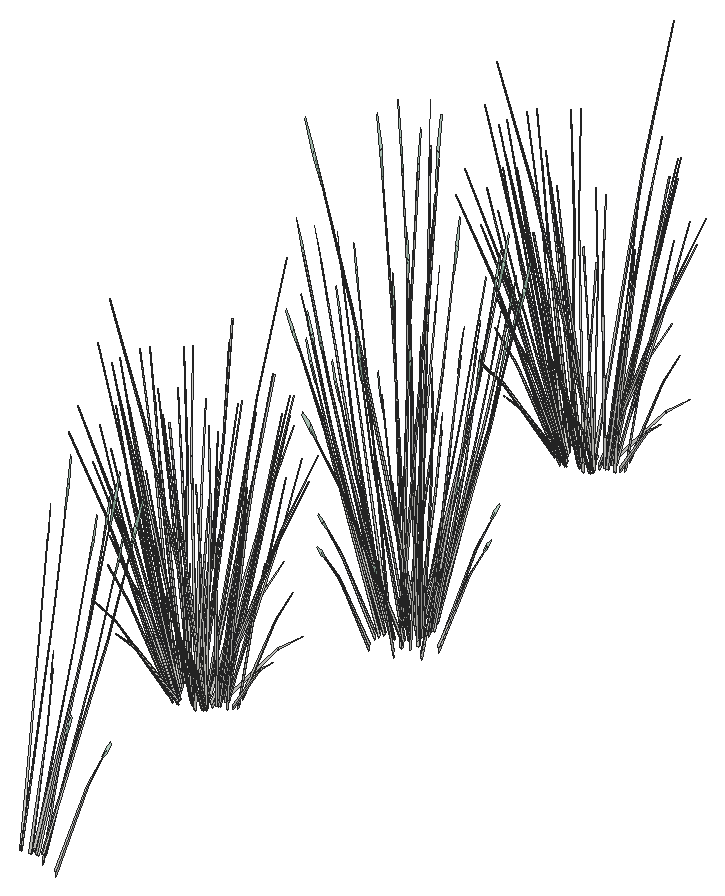
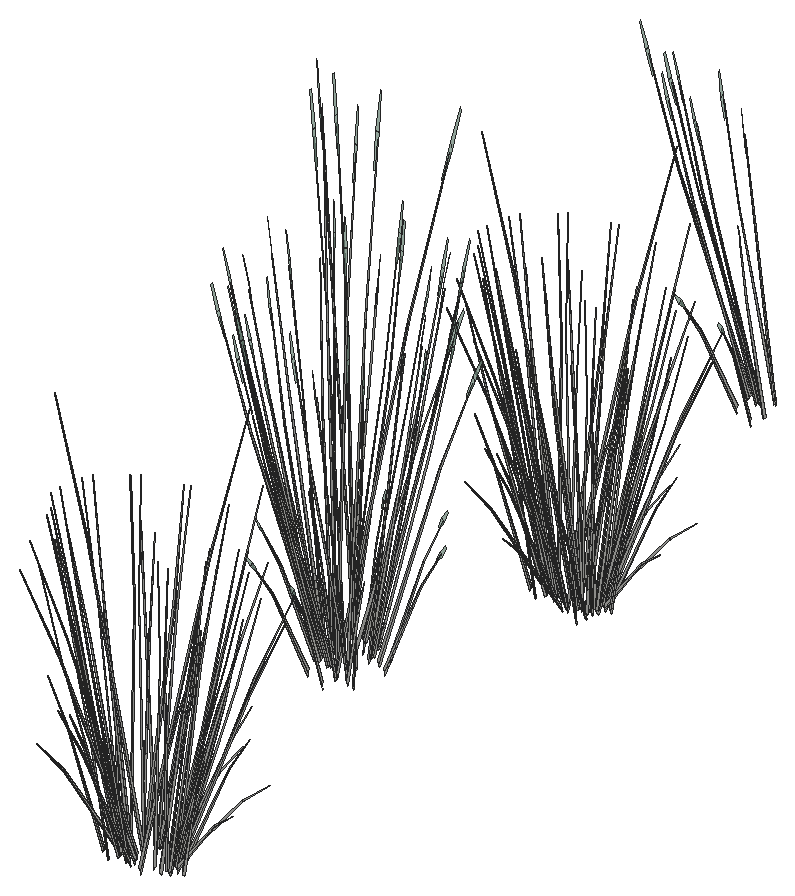
# SketchUp Ruby script. Lengths in inches.
U = 1.inch
M = Sketchup.active_model
def pt(a) = Geom::Point3d.new(a.map { |v| v * U })
def face(e, loops, mat)
  f = e.add_face(loops[0].map { |a| pt(a) })
  loops[1..].each { |l| e.add_face(l.map { |a| pt(a) }).erase! }
  f.material = f.back_material = mat if mat
  f
end
# faces: each face lists its corners as indices into pts; further lists are holes
def faces(e, pts, list, mat = nil) = list.each { |f| face(e, (f[0].is_a?(Array) ? f : [f]).map { |l| l.map { |i| pts[i] } }, mat) }
# xy, xz, yz: faces in a plane at the given z, y or x. An outline is a flat list of corners, or four numbers for a rectangle; further outlines are holes
def ring(l) = l.size == 4 ? [[l[0], l[1]], [l[2], l[1]], [l[2], l[3]], [l[0], l[3]]] : l.each_slice(2).to_a
def flat(e, list, mat, &to3) = list.each { |f| face(e, (f[0].is_a?(Array) ? f : [f]).map { |l| ring(l).map { |u, v| to3.(u, v) } }, mat) }
def xy(e, z, list, mat = nil) = flat(e, list, mat) { |x, y| [x, y, z] }
def xz(e, y, list, mat = nil) = flat(e, list, mat) { |x, z| [x, y, z] }
def yz(e, x, list, mat = nil) = flat(e, list, mat) { |y, z| [x, y, z] }
def lines(e, pts, list) = list.each { |a, b| e.add_line(pt(pts[a]), pt(pts[b])) }
# prism: a flat outline (further loops are holes) pulled along v
def prism(e, loops, v, mat = nil)
  f = face(e, loops, mat); d = Geom::Vector3d.new(v.map { |x| x * U })
  f.pushpull(f.normal.samedirection?(d) ? d.length : -d.length)
end
def box(e, o, s, mat = nil) = prism(e, [[o, [o[0] + s[0], o[1], o[2]], [o[0] + s[0], o[1] + s[1], o[2]], [o[0], o[1] + s[1], o[2]]]], [0, 0, s[2]], mat)
def at(x, y, z, deg = 0) = Geom::Transformation.translation(pt([x, y, z])) * Geom::Transformation.rotation(ORIGIN, Z_AXIS, deg.degrees)
def axes(o, x, y, z) = Geom::Transformation.new([*x, 0, *y, 0, *z, 0, *pt(o).to_a, 1])
def part(name) = M.definitions.add(name)
# library, detail: a bought-in or finely detailed component or shape, given as its bounding box
def library(name, o, s) = part(name).tap { |d| box(d.entities, o, s) }
def detail(e, o, s) = box(e.add_group.entities, o, s)
def put(e, d, t, mat = nil) = e.add_instance(d, t).tap { |i| i.material = mat if mat }
def group(e, t, mat = nil) = e.add_group.tap { |g| g.transformation = t; g.material = mat if mat }.entities
root = M.entities
M.materials.add("LightPink_Translucent").color = [175, 214, 192]
M.materials["LightPink_Translucent"].alpha = 0.75
c1 = part("blade")
p = [[2.15,0.21,22],[0,0.17,0],[0.09,0.45,0],[2.18,0.31,22],[2.29,0.31,22],[0.38,0.45,0],
  [2.48,0.24,33],[2.49,0.24,33],[2.48,0.22,33]]
faces(c1.entities,p,[[0,1,2,3],[4,5,2,3],[6,3,4,7],[8,0,3,6]])
c2 = part("seeds")
p = [[0.3,-0.1,1.38],[-0.01,-0.03,1.59],[-0.01,-0.03,0.03],[0.14,-0.07,-0.07],[0.29,-0.03,3],[0.15,0.01,3.11]]
faces(c2.entities,p,[[0,1,2,3],[1,0,4,5]],"LightPink_Translucent")
c3 = part("blade with seeds")
put(c3.entities,c1,at(0,0,0))
put(c3.entities,c2,axes([2.4,0.25,30.99],[1.5799,-0.05474,1.17369],[-0.12525,1.92788,0.29478],[-0.07173,-0.02425,1.56792]))
c4 = part("blade with seeds\#1")
put(c4.entities,c1,at(0,0,0))
put(root,c3,axes([491.72,471.85,140.75],[0.37435,-0.09148,-0.03177],[0.08606,0.43236,-0.14407],[-0.02373,0.09029,0.47519]))
put(root,c3,axes([494.63,471.6,139.6875],[-0.2267,-0.15919,1.04523],[0.30457,-0.13683,0.76796],[0.07632,0.13148,0.23022]))
put(root,c3,axes([493.78,471.37,141.29],[0.06364,0.41603,-0.32227],[-0.36383,0.10985,0.41605],[0.09772,0.11922,0.79608]))
put(root,c3,axes([493.66,471.04,141.7],[0.35138,0.24965,-0.64651],[-0.24972,0.43748,0.07802],[0.12731,0.14906,0.91455]))
put(root,c3,axes([491.77,471.04,141.29],[-0.27882,0.27194,-0.32227],[-0.26394,-0.31051,0.41605],[-0.04016,0.15777,0.79608]))
put(root,c3,axes([492.92,471.24,141.43],[0.40508,0.12948,-0.465],[-0.13885,0.44393,-0.36018],[0.03714,0.17873,0.88973]))
put(root,c3,axes([492.66,472.36,139.6875],[-0.07352,-0.2953,1.04523],[0.30384,0.139,0.76796],[-0.02079,0.15666,0.23022]))
put(root,c3,axes([492.73,471.52,141.29],[-0.12423,0.3972,-0.32227],[-0.36244,-0.11585,0.41605],[0.03323,0.15992,0.79608]))
put(root,c3,axes([491.95,470.75,141.7],[-0.01072,0.47777,-0.64651],[-0.45152,-0.03209,0.07802],[-0.04765,0.2024,0.91455]))
put(root,c3,axes([492.77,471.16,141.7],[0.19668,0.41997,-0.64651],[-0.40486,0.23405,0.07802],[0.04599,0.20292,0.91455]))
put(root,c4,axes([485.03,499.11,139.9],[0.11364,0.12234,1.40588],[-0.52511,0.103,0.11368],[-0.11868,-0.19206,0.601]))
put(root,c4,axes([485.9,498.29,140.59],[-0.07604,-0.05342,1.43516],[-0.50744,0.03387,-0.22697],[-0.08099,-0.12778,0.1151]))
put(root,c4,axes([488.07,498.68,140.58],[-0.05049,0.0291,1.45516],[-0.49465,-0.09819,-0.1375],[-0.01791,-0.12701,0.25751]))
put(root,c4,axes([488.18,498.95,140.59],[-0.0048,-0.07584,1.43516],[-0.40531,-0.21918,-0.22697],[0.06266,-0.13286,0.1151]))
put(root,c4,axes([486.8,499.32,139.9],[-0.09256,0.13097,1.40588],[-0.38832,-0.27104,0.11368],[0.17518,-0.16893,0.601]))
put(root,c4,axes([486.47,498.93,140.43],[0.14987,-0.29303,-0.29052],[0.43725,0.08547,0.37506],[-0.04009,-0.11798,0.71765]))
put(root,c4,axes([485.375,498.12,140.58],[-0.00927,0.04567,1.45516],[-0.45742,0.16576,-0.1375],[-0.1346,-0.08473,0.25751]))
put(root,c4,axes([486.67,499.12,140.85],[-0.48648,0.17741,-0.09976],[-0.23906,-0.31487,-0.55369],[-0.06419,-0.13269,0.84132]))
put(root,c4,axes([486.53,499,140.6],[0.48986,0.09962,0.39379],[-0.16751,0.3275,0.3247],[-0.02944,-0.12879,0.81485]))
put(root,c4,axes([487.68,499.52,140.85],[-0.54637,-0.01888,-0.09976],[0.01493,-0.35746,-0.55369],[0.03795,-0.13767,0.84132]))
put(root,c4,axes([485.21,499.04,140.43],[-0.07678,-0.30692,-0.29052],[0.43892,-0.08104,0.37506],[-0.11789,-0.08795,0.71765]))
put(root,c4,axes([487.64,499.29,140.43],[0.33637,-0.20062,-0.29052],[0.31842,0.22908,0.37506],[0.04845,-0.11639,0.71765]))
put(root,c4,axes([484.27,499.49,139.9],[0.18466,0.06565,1.40588],[-0.38215,0.27542,0.11368],[-0.23818,-0.12424,0.601]))
put(root,c4,axes([485.5,498.99,141.17],[-0.33178,0.3653,-0.11173],[-0.48049,-0.21045,-0.62013],[-0.16702,-0.10321,0.94228]))
put(root,c4,axes([487.64,499.37,140.6],[0.354,0.25999,0.39379],[-0.37594,0.22422,0.3247],[0.0653,-0.12198,0.81485]))
put(root,c4,axes([484.23,498.88,140.59],[-0.10696,-0.00269,1.43516],[-0.34054,0.26896,-0.22697],[-0.1817,-0.05496,0.1151]))
put(root,c4,axes([488.27,500.22,140.85],[-0.45986,-0.21011,-0.09976],[0.26493,-0.30427,-0.55369],[0.12992,-0.10577,0.84132]))
put(root,c4,axes([489.41,500.13,140.58],[-0.06493,-0.00289,1.45516],[-0.26964,-0.31009,-0.1375],[0.10828,-0.10196,0.25751]))
put(root,c4,axes([486.375,501.37,139.45],[0.4296,0.15365,1.24087],[-0.42086,0.33102,0.4907],[-0.18851,-0.19619,1.04025]))
put(root,c4,axes([484.2,499.58,140.43],[-0.28286,-0.23857,-0.29052],[0.32298,-0.22584,0.37506],[-0.1641,-0.03436,0.71765]))
put(root,c4,axes([488.4,500.01,140.43],[0.43273,-0.05446,-0.29052],[0.11427,0.31131,0.37506],[0.12401,-0.08362,0.71765]))
put(root,c4,axes([488.35,500.08,140.6],[0.12329,0.35069,0.39379],[-0.48364,0.06086,0.3247],[0.14254,-0.08248,0.81485]))
put(root,c4,axes([489.65,500.5,140.59],[0.06898,-0.05804,1.43516],[-0.0883,-0.35603,-0.22697],[0.17309,-0.0675,0.1151]))
put(root,c4,axes([483.82,499.11,140.58],[0.03685,0.03803,1.45516],[-0.17767,0.34183,-0.1375],[-0.17994,0.00247,0.25751]))
put(root,c4,axes([484.52,499.55,140.85],[-0.02662,0.38751,-0.09976],[-0.50399,-0.01059,-0.55369],[-0.19411,-0.02692,0.84132]))
put(root,c4,axes([488.29,501.04,140.85],[-0.25013,-0.34504,-0.09976],[0.44394,-0.16956,-0.55369],[0.18708,-0.04552,0.84132]))
put(root,c4,axes([483.88,500.09,139.9],[0.2062,-0.00863,1.40588],[-0.13679,0.37404,0.11368],[-0.29386,-0.02314,0.601]))
put(root,c4,axes([483.79,500.37,140.6],[0.14045,-0.34743,0.39379],[0.46175,0.1188,0.3247],[-0.18159,0.02088,0.81485]))
put(root,c4,axes([483.7,500.41,140.43],[-0.41315,-0.1063,-0.29052],[0.1205,-0.31012,0.37506],[-0.16634,0.02844,0.71765]))
put(root,c4,axes([488.55,500.9,140.43],[0.41315,0.1063,-0.29052],[-0.1205,0.31012,0.37506],[0.16634,-0.02844,0.71765]))
put(root,c4,axes([487.43,500.52,139.9],[-0.2062,0.00863,1.40588],[0.13679,-0.37404,0.11368],[0.29386,0.02314,0.601]))
put(root,c4,axes([488.46,500.94,140.6],[-0.14045,0.34743,0.39379],[-0.46175,-0.1188,0.3247],[0.18159,-0.02088,0.81485]))
put(root,c4,axes([483.96,500.27,140.85],[0.25013,0.34504,-0.09976],[-0.44394,0.16956,-0.55369],[-0.18708,0.04552,0.84132]))
put(root,c4,axes([489.29,502.07,140.58],[-0.04495,-0.03336,1.45516],[0.09833,-0.35758,-0.1375],[0.17707,-0.02285,0.25751]))
put(root,c4,axes([483.4375,500.61,140.59],[-0.08118,0.04947,1.43516],[0.00691,0.36146,-0.22697],[-0.18608,0.04701,0.1151]))
put(root,c4,axes([488.9,501.77,139.94],[-0.09515,-0.32031,-0.02864],[0.44972,-0.07364,-0.12987],[0.09391,0.02031,0.42837]))
put(root,c4,axes([487.73,501.76,140.85],[0.02662,-0.38751,-0.09976],[0.50399,0.01059,-0.55369],[0.19411,0.02692,0.84132]))
put(root,c4,axes([488.17,501.52,140.59],[0.10664,-0.00644,1.43516],[0.29251,-0.29603,-0.22697],[0.18969,0.03908,0.1151]))
put(root,c4,axes([483.9,501.24,140.6],[-0.12329,-0.35069,0.39379],[0.48364,-0.06086,0.3247],[-0.14254,0.08248,0.81485]))
put(root,c4,axes([483.96,500.75,139.9],[0.17249,-0.0806,1.40588],[0.14522,0.37244,0.11368],[-0.2708,0.08417,0.601]))
put(root,c4,axes([482.53,500.98,140.58],[0.06344,0.01022,1.45516],[0.19627,0.33667,-0.1375],[-0.12987,0.08837,0.25751]))
put(root,c4,axes([483.85,501.3,140.43],[-0.43273,0.05446,-0.29052],[-0.11427,-0.31131,0.37506],[-0.12401,0.08362,0.71765]))
put(root,c4,axes([488.05,501.73,140.43],[0.28286,0.23857,-0.29052],[-0.32298,0.22584,0.37506],[0.1641,0.03436,0.71765]))
put(root,c4,axes([487.94,501.73,140.6],[-0.36656,0.25108,0.39379],[-0.31614,-0.26664,0.3247],[0.17198,0.04631,0.81485]))
put(root,c4,axes([487.07,500.25,140.39],[-0.42958,-0.19798,1.1344],[0.45359,-0.30825,0.48946],[0.1386,0.18577,1.09651]))
put(root,c4,axes([487.04,501.12,139.9],[-0.18466,-0.06565,1.40588],[0.38215,-0.27542,0.11368],[0.23818,0.12424,0.601]))
put(root,c4,axes([483.98,501.09,140.85],[0.45986,0.21011,-0.09976],[-0.26493,0.30427,-0.55369],[-0.12992,0.10577,0.84132]))
put(root,c4,axes([484.6,501,139.9],[0.12417,-0.11708,1.40588],[0.31352,0.31602,0.11368],[-0.21504,0.14392,0.601]))
put(root,c4,axes([486.74,502.18,140.85],[0.29624,-0.32616,-0.09976],[0.42901,0.1879,-0.55369],[0.14913,0.09215,0.84132]))
put(root,c4,axes([486.35,502.45,140.58],[0.00147,-0.04613,1.45516],[0.42603,-0.20353,-0.1375],[0.14798,0.07265,0.25751]))
put(root,c4,axes([484.61,501.95,140.6],[-0.354,-0.25999,0.39379],[0.37594,-0.22422,0.3247],[-0.0653,0.12198,0.81485]))
put(root,c4,axes([486.94,502.23,140.6],[-0.49445,0.08745,0.39379],[-0.08581,-0.34303,0.3247],[0.11629,0.1011,0.81485]))
put(root,c4,axes([484.5,501.28,139.9],[0.09256,-0.13097,1.40588],[0.38832,0.27104,0.11368],[-0.17518,0.16893,0.601]))
put(root,c4,axes([484.61,502.02,140.43],[-0.33637,0.20062,-0.29052],[-0.31842,-0.22908,0.37506],[-0.04845,0.11639,0.71765]))
put(root,c4,axes([483.45,501.96,140.59],[-0.01236,0.0754,1.43516],[0.35069,0.26232,-0.22697],[-0.09181,0.12405,0.1151]))
put(root,c4,axes([484.57,501.79,141.15],[0.54637,0.01888,-0.11073],[-0.01493,0.35746,-0.6146],[-0.03795,0.13767,0.93387]))
put(root,c4,axes([485.58,502.19,140.85],[0.48648,-0.17741,-0.09976],[0.23906,0.31487,-0.55369],[0.06419,0.13269,0.84132]))
put(root,c4,axes([484.94,501.93,140.82],[0.35588,0.25603,-0.4653],[-0.37594,0.22422,-0.36041],[-0.05415,0.13008,0.89031]))
put(root,c4,axes([486.28,501.5,139.9],[-0.11364,-0.12234,1.40588],[0.52511,-0.103,0.11368],[0.11868,0.19206,0.601]))
put(root,c4,axes([485.78,502.38,140.43],[-0.14987,0.29303,-0.29052],[-0.43725,-0.08547,0.37506],[0.04009,0.11798,0.71765]))
put(root,c4,axes([485.35,501.5625,139.9],[-0.01217,-0.14625,1.40588],[0.52737,0.09702,0.11368],[-0.03262,0.20842,0.601]))
put(root,c4,axes([483.41,502.74,140.58],[0.0564,-0.02301,1.45516],[0.46615,0.15302,-0.1375],[-0.01095,0.12741,0.25751]))
put(root,c4,axes([485.47,502.9,140.59],[0.06302,0.06136,1.43516],[0.50855,0.02411,-0.22697],[0.05114,0.13532,0.1151]))
put(root,c4,axes([484.65,502.31,139.48],[0.01092,-0.19671,1.26617],[0.49126,0.1039,0.17497],[-0.04257,0.20964,0.59789]))
put(root,c3,axes([493.37,517.27,140.21],[0.06442,0.13585,1.61128],[-0.4498,0.04685,0.1261],[-0.05969,-0.29426,0.57588]))
put(root,c3,axes([494.09,516.82,141.7],[0.01072,-0.47777,-0.64651],[0.45152,0.03209,0.07802],[0.04765,-0.2024,0.91455]))
put(root,c3,axes([493.3125,516.06,141.29],[0.12423,-0.3972,-0.32227],[0.36244,0.11585,0.41605],[-0.03323,-0.15992,0.79608]))
put(root,c3,axes([493.125,516.33,141.43],[-0.40508,-0.12948,-0.465],[0.13885,-0.44393,-0.36018],[-0.03714,-0.17873,0.88973]))
put(root,c3,axes([494,516.67,141.43],[-0.29499,-0.34704,-0.465],[0.31162,-0.30393,-0.36018],[0.04488,-0.17633,0.88973]))
put(root,c3,axes([491.39,515.45,139.6875],[0.20183,0.19918,1.04523],[-0.31952,0.0786,0.76796],[-0.05721,-0.14394,0.23022]))
put(root,c3,axes([494.28,516.54,141.29],[0.27882,-0.27194,-0.32227],[0.26394,0.31051,0.41605],[0.04016,-0.15777,0.79608]))
put(root,c3,axes([492.27,516.2,141.29],[-0.06364,-0.41603,-0.32227],[0.36383,-0.10985,0.41605],[-0.09772,-0.11922,0.79608]))
put(root,c3,axes([493.61,515.88,139.6875],[0.03187,0.30513,1.04523],[-0.28077,-0.19355,0.76796],[0.04212,-0.15079,0.23022]))
put(root,c3,axes([492.22,516.54,141.43],[-0.40663,0.12278,-0.465],[-0.07113,-0.46497,-0.36018],[-0.10922,-0.13325,0.88973]))
put(root,c3,axes([494.625,517.65,141.7],[0.21525,-0.40754,-0.64651],[0.37719,0.28963,0.07802],[0.12852,-0.14765,0.91455]))
put(root,c3,axes([494.61,517.46,141.43],[-0.10586,-0.47162,-0.465],[0.4009,-0.0825,-0.36018],[0.11489,-0.12667,0.88973]))
put(root,c3,axes([494.91,517.51,141.29],[0.3587,-0.07382,-0.32227],[0.09472,0.42197,0.41605],[0.10279,-0.11334,0.79608]))
put(root,c3,axes([491.42,516.93,141.29],[-0.23447,-0.32338,-0.32227],[0.26773,-0.30612,0.41605],[-0.13603,-0.04658,0.79608]))
put(root,c3,axes([492.19,518.63,140.2],[-0.17958,0.41302,1.37647],[-0.38687,-0.40462,0.54432],[0.22929,-0.18124,1.15394]))
put(root,c3,axes([495.45,517.05,139.6875],[-0.155,0.24931,1.04523],[-0.09317,-0.36309,0.76796],[0.11912,-0.07769,0.23022]))
put(root,c3,axes([491.67,517.15,142.03],[-0.41193,-0.01244,-0.71763],[0.02767,-0.52368,0.0866],[-0.17451,-0.05527,1.01516]))
put(root,c3,axes([490.51,517.14,139.6875],[0.2648,-0.01237,1.04523],[-0.18886,0.30908,0.76796],[-0.12621,-0.06079,0.23022]))
put(root,c3,axes([491.09,516.97,140.23],[0.22989,0.0105,1.40454],[-0.12143,0.4723,0.19409],[-0.24501,-0.04092,0.66323]))
put(root,c3,axes([491.54,517.26,141.72],[-0.29922,0.34214,-0.51615],[-0.26205,-0.36143,-0.3998],[-0.15203,-0.05206,0.9876]))
put(root,c3,axes([493.05,519.27,139.76],[0.4193,-0.01306,1.28558],[-0.10869,0.59089,0.54432],[-0.22943,-0.13975,1.21348]))
put(root,c3,axes([494.8,518.51,141.43],[0.11164,-0.46982,-0.465],[0.38276,0.16104,-0.36018],[0.1541,-0.04308,0.88973]))
put(root,c3,axes([492.79,517.92,139.64],[-0.40128,-0.23189,0.40713],[0.19312,-0.48183,-0.19594],[0.0925,0,1.30716]))
put(root,c3,axes([494.73,518.68,141.7],[0.3621,-0.22811,-0.64651],[0.2018,0.46957,0.07802],[0.17496,-0.05334,0.91455]))
put(root,c3,axes([492.61,519.04,139.64],[0.02749,0.519,0.40713],[-0.45634,0.04694,-0.19594],[-0.04625,-0.09291,1.30716]))
put(root,c3,axes([495.04,518.73,141.29],[0.34247,0.14409,-0.32227],[-0.09989,0.42037,0.41605],[0.13788,-0.03855,0.79608]))
put(root,c3,axes([491.01,518.06,141.29],[-0.34247,-0.14409,-0.32227],[0.09989,-0.42037,0.41605],[-0.13788,0.03855,0.79608]))
put(root,c3,axes([493.35,518.04,139.64],[-0.02749,-0.519,0.40713],[0.45634,-0.04694,-0.19594],[0.04625,0.09291,1.30716]))
put(root,c3,axes([491.32,518.1,141.7],[-0.3621,0.22811,-0.64651],[-0.2018,-0.46957,0.07802],[-0.17496,0.05334,0.91455]))
put(root,c3,axes([495.76,518.8,139.6875],[-0.25968,0.06131,1.04523],[0.14383,-0.34012,0.76796],[0.13297,0.0366,0.23022]))
put(root,c3,axes([493.17,519.16,139.64],[0.40128,0.23189,0.40713],[-0.19312,0.48183,-0.19594],[-0.0925,0,1.30716]))
put(root,c3,axes([491.25,518.27,141.43],[-0.11164,0.46982,-0.465],[-0.38276,-0.16104,-0.36018],[-0.1541,0.04308,0.88973]))
put(root,c3,axes([493.54,518.66,139.64],[0.37379,-0.28711,0.40713],[0.26322,0.43489,-0.19594],[-0.04625,0.09291,1.30716]))
put(root,c3,axes([494.51,519.53,141.43],[0.29922,-0.34214,-0.465],[0.26205,0.36143,-0.36018],[0.15203,0.05206,0.88973]))
put(root,c3,axes([494.375,519.63,141.7],[0.41193,0.01244,-0.64651],[-0.02767,0.52368,0.07802],[0.17451,0.05527,0.91455]))
put(root,c3,axes([494.62,519.85,141.29],[0.23447,0.32338,-0.32227],[-0.26773,0.30612,0.41605],[0.13603,0.04658,0.79608]))
put(root,c3,axes([491.61,519.93,139.6875],[0.12805,-0.2691,1.04523],[0.13011,0.34747,0.76796],[-0.11021,0.09372,0.23022]))
put(root,c3,axes([491.02,519.97,139.6],[0.01397,-0.30649,0.95605],[0.29664,0.2024,0.52785],[-0.10539,0.12108,0.74993]))
put(root,c3,axes([491.43,519.32,141.43],[0.10586,0.47162,-0.465],[-0.4009,0.0825,-0.36018],[-0.11489,0.12667,0.88973]))
put(root,c3,axes([493.82,520.24,141.43],[0.40663,-0.12278,-0.465],[0.07113,0.46497,-0.36018],[0.10922,0.13325,0.88973]))
put(root,c3,axes([491.72,521.05,140.75],[0.37435,-0.09148,-0.03177],[0.08606,0.43236,-0.14407],[-0.02373,0.09029,0.47519]))
put(root,c3,axes([494.63,520.81,139.6875],[-0.2267,-0.15919,1.04523],[0.30457,-0.13683,0.76796],[0.07632,0.13148,0.23022]))
put(root,c3,axes([493.78,520.58,141.29],[0.06364,0.41603,-0.32227],[-0.36383,0.10985,0.41605],[0.09772,0.11922,0.79608]))
put(root,c3,axes([493.66,520.25,141.7],[0.35138,0.24965,-0.64651],[-0.24972,0.43748,0.07802],[0.12731,0.14906,0.91455]))
put(root,c3,axes([491.77,520.25,141.29],[-0.27882,0.27194,-0.32227],[-0.26394,-0.31051,0.41605],[-0.04016,0.15777,0.79608]))
put(root,c3,axes([492.92,520.45,141.43],[0.40508,0.12948,-0.465],[-0.13885,0.44393,-0.36018],[0.03714,0.17873,0.88973]))
put(root,c3,axes([492.66,521.57,139.6875],[-0.07352,-0.2953,1.04523],[0.30384,0.139,0.76796],[-0.02079,0.15666,0.23022]))
put(root,c3,axes([492.73,520.73,141.29],[-0.12423,0.3972,-0.32227],[-0.36244,-0.11585,0.41605],[0.03323,0.15992,0.79608]))
put(root,c3,axes([491.95,519.96,141.7],[-0.01072,0.47777,-0.64651],[-0.45152,-0.03209,0.07802],[-0.04765,0.2024,0.91455]))
put(root,c3,axes([492.77,520.37,141.7],[0.19668,0.41997,-0.64651],[-0.40486,0.23405,0.07802],[0.04599,0.20292,0.91455]))
put(root,c4,axes([485.03,548.15,139.9],[0.11364,0.12234,1.40588],[-0.52511,0.103,0.11368],[-0.11868,-0.19206,0.601]))
put(root,c4,axes([485.9,547.34,140.59],[-0.07604,-0.05342,1.43516],[-0.50744,0.03387,-0.22697],[-0.08099,-0.12778,0.1151]))
put(root,c4,axes([488.07,547.73,140.58],[-0.05049,0.0291,1.45516],[-0.49465,-0.09819,-0.1375],[-0.01791,-0.12701,0.25751]))
put(root,c4,axes([488.18,548,140.59],[-0.0048,-0.07584,1.43516],[-0.40531,-0.21918,-0.22697],[0.06266,-0.13286,0.1151]))
put(root,c4,axes([486.8,548.37,139.9],[-0.09256,0.13097,1.40588],[-0.38832,-0.27104,0.11368],[0.17518,-0.16893,0.601]))
put(root,c4,axes([486.47,547.98,140.43],[0.14987,-0.29303,-0.29052],[0.43725,0.08547,0.37506],[-0.04009,-0.11798,0.71765]))
put(root,c4,axes([485.375,547.17,140.58],[-0.00927,0.04567,1.45516],[-0.45742,0.16576,-0.1375],[-0.1346,-0.08473,0.25751]))
put(root,c4,axes([486.67,548.17,140.85],[-0.48648,0.17741,-0.09976],[-0.23906,-0.31487,-0.55369],[-0.06419,-0.13269,0.84132]))
put(root,c4,axes([486.53,548.05,140.6],[0.48986,0.09962,0.39379],[-0.16751,0.3275,0.3247],[-0.02944,-0.12879,0.81485]))
put(root,c4,axes([487.68,548.57,140.85],[-0.54637,-0.01888,-0.09976],[0.01493,-0.35746,-0.55369],[0.03795,-0.13767,0.84132]))
put(root,c4,axes([485.21,548.09,140.43],[-0.07678,-0.30692,-0.29052],[0.43892,-0.08104,0.37506],[-0.11789,-0.08795,0.71765]))
put(root,c4,axes([487.64,548.34,140.43],[0.33637,-0.20062,-0.29052],[0.31842,0.22908,0.37506],[0.04845,-0.11639,0.71765]))
put(root,c4,axes([484.27,548.54,139.9],[0.18466,0.06565,1.40588],[-0.38215,0.27542,0.11368],[-0.23818,-0.12424,0.601]))
put(root,c4,axes([485.5,548.04,141.17],[-0.33178,0.3653,-0.11173],[-0.48049,-0.21045,-0.62013],[-0.16702,-0.10321,0.94228]))
put(root,c4,axes([487.64,548.41,140.6],[0.354,0.25999,0.39379],[-0.37594,0.22422,0.3247],[0.0653,-0.12198,0.81485]))
put(root,c4,axes([484.23,547.93,140.59],[-0.10696,-0.00269,1.43516],[-0.34054,0.26896,-0.22697],[-0.1817,-0.05496,0.1151]))
put(root,c4,axes([488.27,549.27,140.85],[-0.45986,-0.21011,-0.09976],[0.26493,-0.30427,-0.55369],[0.12992,-0.10577,0.84132]))
put(root,c4,axes([489.41,549.18,140.58],[-0.06493,-0.00289,1.45516],[-0.26964,-0.31009,-0.1375],[0.10828,-0.10196,0.25751]))
put(root,c4,axes([486.375,550.42,139.45],[0.4296,0.15365,1.24087],[-0.42086,0.33102,0.4907],[-0.18851,-0.19619,1.04025]))
put(root,c4,axes([484.2,548.63,140.43],[-0.28286,-0.23857,-0.29052],[0.32298,-0.22584,0.37506],[-0.1641,-0.03436,0.71765]))
put(root,c4,axes([488.4,549.06,140.43],[0.43273,-0.05446,-0.29052],[0.11427,0.31131,0.37506],[0.12401,-0.08362,0.71765]))
put(root,c4,axes([488.35,549.125,140.6],[0.12329,0.35069,0.39379],[-0.48364,0.06086,0.3247],[0.14254,-0.08248,0.81485]))
put(root,c4,axes([489.65,549.55,140.59],[0.06898,-0.05804,1.43516],[-0.0883,-0.35603,-0.22697],[0.17309,-0.0675,0.1151]))
put(root,c4,axes([483.82,548.16,140.58],[0.03685,0.03803,1.45516],[-0.17767,0.34183,-0.1375],[-0.17994,0.00247,0.25751]))
put(root,c4,axes([484.52,548.6,140.85],[-0.02662,0.38751,-0.09976],[-0.50399,-0.01059,-0.55369],[-0.19411,-0.02692,0.84132]))
put(root,c4,axes([488.29,550.09,140.85],[-0.25013,-0.34504,-0.09976],[0.44394,-0.16956,-0.55369],[0.18708,-0.04552,0.84132]))
put(root,c4,axes([483.88,549.14,139.9],[0.2062,-0.00863,1.40588],[-0.13679,0.37404,0.11368],[-0.29386,-0.02314,0.601]))
put(root,c4,axes([483.79,549.42,140.6],[0.14045,-0.34743,0.39379],[0.46175,0.1188,0.3247],[-0.18159,0.02088,0.81485]))
put(root,c4,axes([483.7,549.46,140.43],[-0.41315,-0.1063,-0.29052],[0.1205,-0.31012,0.37506],[-0.16634,0.02844,0.71765]))
put(root,c4,axes([488.55,549.95,140.43],[0.41315,0.1063,-0.29052],[-0.1205,0.31012,0.37506],[0.16634,-0.02844,0.71765]))
put(root,c4,axes([487.43,549.57,139.9],[-0.2062,0.00863,1.40588],[0.13679,-0.37404,0.11368],[0.29386,0.02314,0.601]))
put(root,c4,axes([488.46,549.99,140.6],[-0.14045,0.34743,0.39379],[-0.46175,-0.1188,0.3247],[0.18159,-0.02088,0.81485]))
put(root,c4,axes([483.96,549.32,140.85],[0.25013,0.34504,-0.09976],[-0.44394,0.16956,-0.55369],[-0.18708,0.04552,0.84132]))
put(root,c4,axes([489.29,551.11,140.58],[-0.04495,-0.03336,1.45516],[0.09833,-0.35758,-0.1375],[0.17707,-0.02285,0.25751]))
put(root,c4,axes([483.4375,549.66,140.59],[-0.08118,0.04947,1.43516],[0.00691,0.36146,-0.22697],[-0.18608,0.04701,0.1151]))
put(root,c4,axes([488.9,550.82,139.94],[-0.09515,-0.32031,-0.02864],[0.44972,-0.07364,-0.12987],[0.09391,0.02031,0.42837]))
put(root,c4,axes([487.73,550.81,140.85],[0.02662,-0.38751,-0.09976],[0.50399,0.01059,-0.55369],[0.19411,0.02692,0.84132]))
put(root,c4,axes([488.17,550.57,140.59],[0.10664,-0.00644,1.43516],[0.29251,-0.29603,-0.22697],[0.18969,0.03908,0.1151]))
put(root,c4,axes([483.9,550.28,140.6],[-0.12329,-0.35069,0.39379],[0.48364,-0.06086,0.3247],[-0.14254,0.08248,0.81485]))
put(root,c4,axes([483.96,549.79,139.9],[0.17249,-0.0806,1.40588],[0.14522,0.37244,0.11368],[-0.2708,0.08417,0.601]))
put(root,c4,axes([482.53,550.03,140.58],[0.06344,0.01022,1.45516],[0.19627,0.33667,-0.1375],[-0.12987,0.08837,0.25751]))
put(root,c4,axes([483.85,550.35,140.43],[-0.43273,0.05446,-0.29052],[-0.11427,-0.31131,0.37506],[-0.12401,0.08362,0.71765]))
put(root,c4,axes([488.05,550.78,140.43],[0.28286,0.23857,-0.29052],[-0.32298,0.22584,0.37506],[0.1641,0.03436,0.71765]))
put(root,c4,axes([487.94,550.78,140.6],[-0.36656,0.25108,0.39379],[-0.31614,-0.26664,0.3247],[0.17198,0.04631,0.81485]))
put(root,c4,axes([487.07,549.3,140.39],[-0.42958,-0.19798,1.1344],[0.45359,-0.30825,0.48946],[0.1386,0.18577,1.09651]))
put(root,c4,axes([487.04,550.17,139.9],[-0.18466,-0.06565,1.40588],[0.38215,-0.27542,0.11368],[0.23818,0.12424,0.601]))
put(root,c4,axes([483.98,550.14,140.85],[0.45986,0.21011,-0.09976],[-0.26493,0.30427,-0.55369],[-0.12992,0.10577,0.84132]))
put(root,c4,axes([484.6,550.05,139.9],[0.12417,-0.11708,1.40588],[0.31352,0.31602,0.11368],[-0.21504,0.14392,0.601]))
put(root,c4,axes([486.74,551.23,140.85],[0.29624,-0.32616,-0.09976],[0.42901,0.1879,-0.55369],[0.14913,0.09215,0.84132]))
put(root,c4,axes([486.35,551.5,140.58],[0.00147,-0.04613,1.45516],[0.42603,-0.20353,-0.1375],[0.14798,0.07265,0.25751]))
put(root,c4,axes([484.61,550.99,140.6],[-0.354,-0.25999,0.39379],[0.37594,-0.22422,0.3247],[-0.0653,0.12198,0.81485]))
put(root,c4,axes([486.94,551.28,140.6],[-0.49445,0.08745,0.39379],[-0.08581,-0.34303,0.3247],[0.11629,0.1011,0.81485]))
